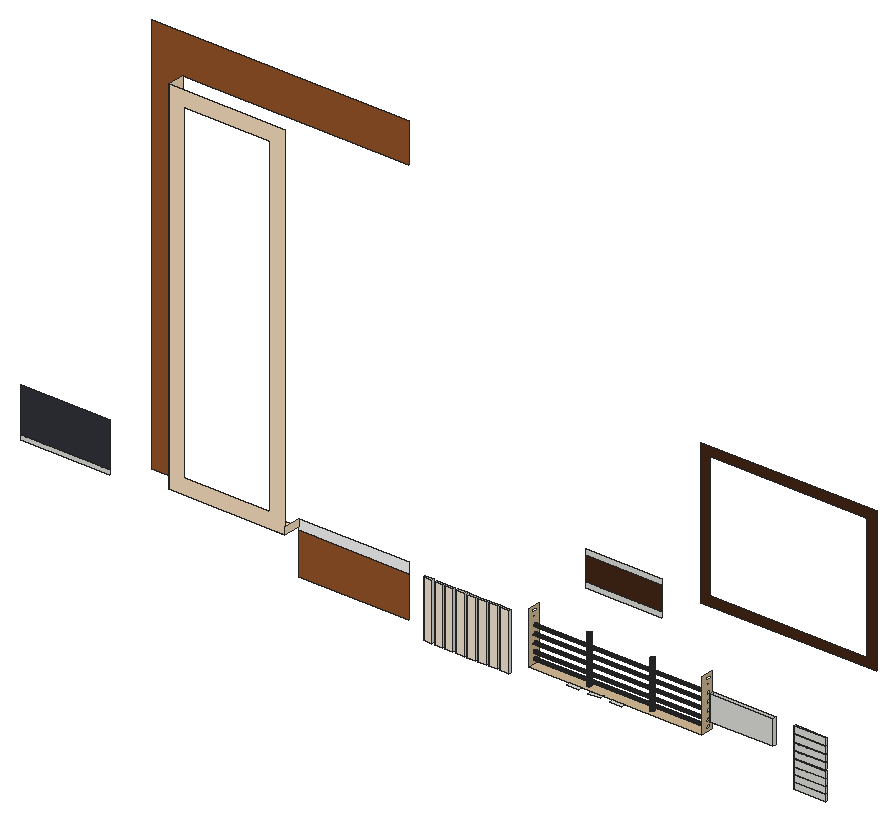
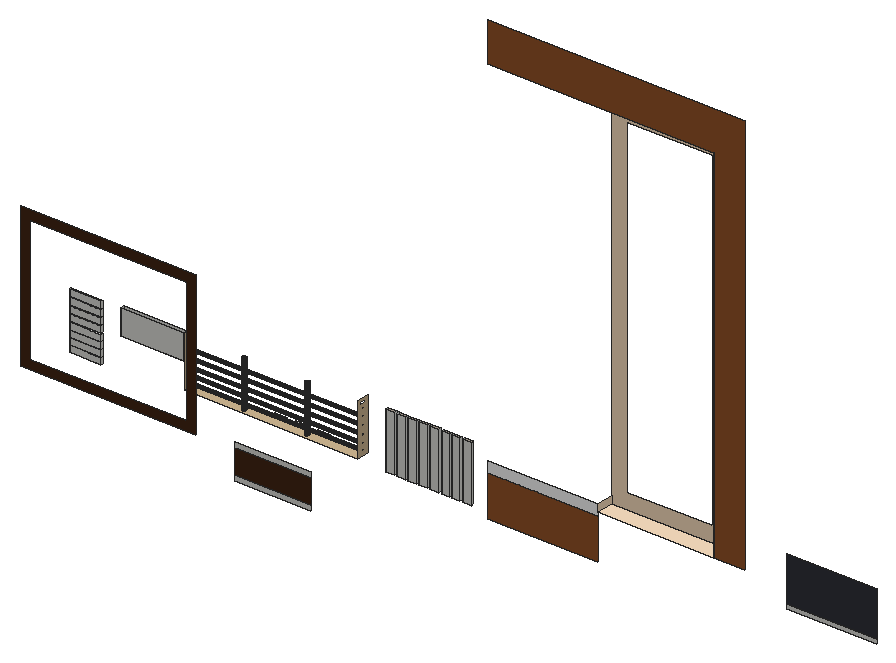
# SketchUp Ruby script. Lengths in inches.
U = 1.inch
M = Sketchup.active_model
def pt(a) = Geom::Point3d.new(a.map { |v| v * U })
def face(e, loops, mat)
  f = e.add_face(loops[0].map { |a| pt(a) })
  loops[1..].each { |l| e.add_face(l.map { |a| pt(a) }).erase! }
  f.material = f.back_material = mat if mat
  f
end
# faces: each face lists its corners as indices into pts; further lists are holes
def faces(e, pts, list, mat = nil) = list.each { |f| face(e, (f[0].is_a?(Array) ? f : [f]).map { |l| l.map { |i| pts[i] } }, mat) }
# xy, xz, yz: faces in a plane at the given z, y or x. An outline is a flat list of corners, or four numbers for a rectangle; further outlines are holes
def ring(l) = l.size == 4 ? [[l[0], l[1]], [l[2], l[1]], [l[2], l[3]], [l[0], l[3]]] : l.each_slice(2).to_a
def flat(e, list, mat, &to3) = list.each { |f| face(e, (f[0].is_a?(Array) ? f : [f]).map { |l| ring(l).map { |u, v| to3.(u, v) } }, mat) }
def xy(e, z, list, mat = nil) = flat(e, list, mat) { |x, y| [x, y, z] }
def xz(e, y, list, mat = nil) = flat(e, list, mat) { |x, z| [x, y, z] }
def yz(e, x, list, mat = nil) = flat(e, list, mat) { |y, z| [x, y, z] }
def lines(e, pts, list) = list.each { |a, b| e.add_line(pt(pts[a]), pt(pts[b])) }
# prism: a flat outline (further loops are holes) pulled along v
def prism(e, loops, v, mat = nil)
  f = face(e, loops, mat); d = Geom::Vector3d.new(v.map { |x| x * U })
  f.pushpull(f.normal.samedirection?(d) ? d.length : -d.length)
end
def box(e, o, s, mat = nil) = prism(e, [[o, [o[0] + s[0], o[1], o[2]], [o[0] + s[0], o[1] + s[1], o[2]], [o[0], o[1] + s[1], o[2]]]], [0, 0, s[2]], mat)
def at(x, y, z, deg = 0) = Geom::Transformation.translation(pt([x, y, z])) * Geom::Transformation.rotation(ORIGIN, Z_AXIS, deg.degrees)
def axes(o, x, y, z) = Geom::Transformation.new([*x, 0, *y, 0, *z, 0, *pt(o).to_a, 1])
def part(name) = M.definitions.add(name)
# library, detail: a bought-in or finely detailed component or shape, given as its bounding box
def library(name, o, s) = part(name).tap { |d| box(d.entities, o, s) }
def detail(e, o, s) = box(e.add_group.entities, o, s)
def put(e, d, t, mat = nil) = e.add_instance(d, t).tap { |i| i.material = mat if mat }
def group(e, t, mat = nil) = e.add_group.tap { |g| g.transformation = t; g.material = mat if mat }.entities
root = M.entities
M.materials.add("[0012_Bisque]").color = [255, 228, 196]
M.materials.add("[0028_AntiqueWhite]").color = [250, 235, 215]
M.materials.add("[Color M00]").color = [255, 255, 255]
M.materials.add("[Color M08]").color = [30, 30, 30]
M.materials.add("[Formica Beige]").color = [211, 187, 149]
M.materials.add("[Formica Laminate Dark]").color = [50, 53, 60]
M.materials.add("[Wood Cherry Original]").color = [152, 86, 42]
M.materials.add("[Wood Veneer 01]").color = [68, 40, 21]
box(root,[409.2,39.8,138.47],[15.5,0.87,3.18])
box(root,[409.2,39.8,141.72],[15.5,0.87,3.18])
box(root,[409.2,39.8,145.15],[15.5,0.87,3.19])
box(root,[409.2,39.8,148.53],[15.5,0.87,3.19])
box(root,[409.2,39.8,152.34],[15.5,0.87,3.19])
box(root,[409.2,39.8,155.84],[15.5,0.87,3.19])
box(root,[409.2,39.8,159.47],[15.5,0.87,3.18])
xy(root,140.39,[[227.93,39.48,232.05,40.67],[233.37,39.48,237.49,40.67],[238.43,39.48,242.55,40.67],[244.05,39.48,248.18,40.67],[249.43,39.48,253.55,40.67],
  [254.74,39.48,258.87,40.67],[260.12,39.48,264.24,40.67],[265.49,39.48,269.62,40.67]])
xy(root,145.875,[[298.64,38.8,304.69,40.67],[309.14,38.8,315.19,40.67],[319.64,38.8,325.69,40.67],[336.54,43.14,336.28,43.17,336.04,43.27,335.83,43.43,335.67,43.64,335.57,43.88,335.54,44.14,335.57,44.4,335.67,44.64,335.83,44.85,336.04,45.01,336.28,45.11,336.54,45.14,336.79,45.11,337.04,45.01,337.24,44.85,337.4,44.64,337.5,44.4,337.54,44.14,337.5,43.88,337.4,43.64,337.24,43.43,337.04,43.27,336.79,43.17]])
xy(root,145.875,[[[278.51,40.67,363.63,46.73],[305.54,43.14,305.28,43.17,305.04,43.27,304.83,43.43,304.67,43.64,304.57,43.88,304.54,44.14,304.57,44.4,304.67,44.64,304.83,44.85,305.04,45.01,305.28,45.11,305.54,45.14,305.79,45.11,306.04,45.01,306.24,44.85,306.4,44.64,306.5,44.4,306.54,44.14,306.5,43.88,306.4,43.64,306.24,43.43,306.04,43.27,305.79,43.17],[336.54,43.14,336.28,43.17,336.04,43.27,335.83,43.43,335.67,43.64,335.57,43.88,335.54,44.14,335.57,44.4,335.67,44.64,335.83,44.85,336.04,45.01,336.28,45.11,336.54,45.14,336.79,45.11,337.04,45.01,337.24,44.85,337.4,44.64,337.5,44.4,337.54,44.14,337.5,43.88,337.4,43.64,337.24,43.43,337.04,43.27,336.79,43.17]]],"[Formica Beige]")
xy(root,154.46,[[368.61,38.8,399.74,40.67]])
xy(root,163.09,[[409.2,39.8,424.7,40.67]])
xy(root,163.67,[[104.08,38.36,161.14,46.73]],"[0012_Bisque]")
xz(root,38.36,[[[104.08,163.67,161.14,341.36],[111.55,171.14,153.67,333.89]]],"[0012_Bisque]")
xz(root,38.8,[[368.61,154.46,399.74,166.58]])
xz(root,39.48,[[227.93,140.39,232.05,168.02],[233.37,140.39,237.49,168.02],[238.43,140.39,242.55,168.02],[244.05,140.39,248.18,168.02],[249.43,140.39,253.55,168.02],
  [254.74,140.39,258.87,168.02],[260.12,140.39,264.24,168.02],[265.49,140.39,269.62,168.02]],"[0028_AntiqueWhite]")
xz(root,39.8,[[409.2,163.09,424.7,166.28]])
xz(root,40.67,[[227.93,140.39,232.05,168.02],[233.37,140.39,237.49,168.02],[238.43,140.39,242.55,168.02],[244.05,140.39,248.18,168.02],[249.43,140.39,253.55,168.02],
  [254.74,140.39,258.87,168.02],[260.12,140.39,264.24,168.02],[265.49,140.39,269.62,168.02],[368.61,154.46,399.74,166.58],[409.2,163.09,424.7,166.28]])
xz(root,46.73,[[24.6875,153.73,68.38,156.02]])
xz(root,46.73,[[161.14,161.98,215,167.14]],"[Color M00]")
xz(root,46.73,[[24.6875,156.02,68.38,177.73]],"[Formica Laminate Dark]")
xz(root,46.73,[[161.14,141.51,215,161.98],[89.06,163.67,104.08,163.67,104.08,341.36,215,341.36,215,360.6,89.06,360.6]],"[Wood Cherry Original]")
xz(root,96.17,[[262.03,150.42,299.47,153.01],[262.03,164.92,299.47,167.51]])
xz(root,96.17,[[262.03,153.01,299.47,164.92],[[318.53,163.84,404.47,234.09],[323.03,168.34,399.97,229.59]]],"[Wood Veneer 01]")
yz(root,104.08,[[38.36,163.67,46.73,341.36]],"[0012_Bisque]")
yz(root,161.14,[[38.36,163.67,46.73,167.14]],"[0012_Bisque]")
yz(root,227.93,[[39.48,140.39,40.67,168.02]])
yz(root,232.05,[[39.48,140.39,40.67,168.02]])
yz(root,233.37,[[39.48,140.39,40.67,168.02]])
yz(root,237.49,[[39.48,140.39,40.67,168.02]])
yz(root,238.43,[[39.48,140.39,40.67,168.02]])
yz(root,242.55,[[39.48,140.39,40.67,168.02]])
yz(root,244.05,[[39.48,140.39,40.67,168.02]])
yz(root,248.18,[[39.48,140.39,40.67,168.02]])
yz(root,249.43,[[39.48,140.39,40.67,168.02]])
yz(root,253.55,[[39.48,140.39,40.67,168.02]])
yz(root,254.74,[[39.48,140.39,40.67,168.02]])
yz(root,258.87,[[39.48,140.39,40.67,168.02]])
yz(root,260.12,[[39.48,140.39,40.67,168.02]])
yz(root,264.24,[[39.48,140.39,40.67,168.02]])
yz(root,265.49,[[39.48,140.39,40.67,168.02]])
yz(root,269.62,[[39.48,140.39,40.67,168.02]])
yz(root,278.51,[[[40.67,145.875,46.73,171.25],[42.95,168.7,45.58,170.07],[43.9,166.34,43.74,166.37,43.59,166.4375,43.47,166.54,43.37,166.68,43.3125,166.83,43.3,166.99,43.33,167.15,43.39,167.3,43.5,167.43,43.63,167.52,43.78,167.58,43.94,167.59,44.11,167.57,44.25,167.5,44.38,167.4,44.47,167.26,44.53,167.11,44.55,166.95,44.52,166.79,44.45,166.64,44.35,166.51,44.22,166.42,44.06,166.36],[43.9,162.53,43.74,162.56,43.59,162.625,43.47,162.73,43.37,162.86,43.3125,163.02,43.3,163.18,43.33,163.34,43.39,163.49,43.5,163.61,43.63,163.71,43.78,163.77,43.94,163.78,44.11,163.76,44.25,163.6875,44.38,163.58,44.47,163.45,44.53,163.3,44.55,163.14,44.52,162.97,44.45,162.83,44.35,162.7,44.22,162.61,44.06,162.55],[43.9,158.53,43.74,158.56,43.59,158.625,43.47,158.73,43.37,158.86,43.3125,159.02,43.3,159.18,43.33,159.34,43.39,159.49,43.5,159.61,43.63,159.71,43.78,159.77,43.94,159.78,44.11,159.76,44.25,159.6875,44.38,159.58,44.47,159.45,44.53,159.3,44.55,159.14,44.52,158.97,44.45,158.83,44.35,158.7,44.22,158.61,44.06,158.55],[43.9,154.53,43.74,154.56,43.59,154.625,43.47,154.73,43.37,154.86,43.3125,155.02,43.3,155.18,43.33,155.34,43.39,155.49,43.5,155.61,43.63,155.71,43.78,155.77,43.94,155.78,44.11,155.76,44.25,155.6875,44.38,155.58,44.47,155.45,44.53,155.3,44.55,155.14,44.52,154.97,44.45,154.83,44.35,154.7,44.22,154.61,44.06,154.55],[43.9,147.66,43.74,147.68,43.59,147.75,43.47,147.86,43.37,147.99,43.3125,148.14,43.3,148.3,43.33,148.46,43.39,148.61,43.5,148.74,43.63,148.83,43.78,148.89,43.94,148.91,44.11,148.88,44.25,148.8125,44.38,148.71,44.47,148.58,44.53,148.42,44.55,148.26,44.52,148.1,44.45,147.95,44.35,147.83,44.22,147.73,44.06,147.67],[43.9,150.84,43.74,150.87,43.59,150.9375,43.47,151.04,43.37,151.18,43.3125,151.33,43.3,151.49,43.33,151.65,43.39,151.8,43.5,151.93,43.63,152.02,43.78,152.08,43.94,152.09,44.11,152.07,44.25,152,44.38,151.9,44.47,151.76,44.53,151.61,44.55,151.45,44.52,151.29,44.45,151.14,44.35,151.01,44.22,150.92,44.06,150.86]]],"[Formica Beige]")
yz(root,363.63,[[43.9,147.66,44.06,147.67,44.22,147.73,44.35,147.83,44.45,147.95,44.52,148.1,44.55,148.26,44.53,148.42,44.47,148.58,44.38,148.71,44.25,148.8125,44.11,148.88,43.94,148.91,43.78,148.89,43.63,148.83,43.5,148.74,43.39,148.61,43.33,148.46,43.3,148.3,43.3125,148.14,43.37,147.99,43.47,147.86,43.59,147.75,43.74,147.68],[43.9,150.84,44.06,150.86,44.22,150.92,44.35,151.01,44.45,151.14,44.52,151.29,44.55,151.45,44.53,151.61,44.47,151.76,44.38,151.9,44.25,152,44.11,152.07,43.94,152.09,43.78,152.08,43.63,152.02,43.5,151.93,43.39,151.8,43.33,151.65,43.3,151.49,43.3125,151.33,43.37,151.18,43.47,151.04,43.59,150.9375,43.74,150.87],[43.9,154.53,44.06,154.55,44.22,154.61,44.35,154.7,44.45,154.83,44.52,154.97,44.55,155.14,44.53,155.3,44.47,155.45,44.38,155.58,44.25,155.6875,44.11,155.76,43.94,155.78,43.78,155.77,43.63,155.71,43.5,155.61,43.39,155.49,43.33,155.34,43.3,155.18,43.3125,155.02,43.37,154.86,43.47,154.73,43.59,154.625,43.74,154.56],[43.9,158.53,44.06,158.55,44.22,158.61,44.35,158.7,44.45,158.83,44.52,158.97,44.55,159.14,44.53,159.3,44.47,159.45,44.38,159.58,44.25,159.6875,44.11,159.76,43.94,159.78,43.78,159.77,43.63,159.71,43.5,159.61,43.39,159.49,43.33,159.34,43.3,159.18,43.3125,159.02,43.37,158.86,43.47,158.73,43.59,158.625,43.74,158.56],[43.9,162.53,44.06,162.55,44.22,162.61,44.35,162.7,44.45,162.83,44.52,162.97,44.55,163.14,44.53,163.3,44.47,163.45,44.38,163.58,44.25,163.6875,44.11,163.76,43.94,163.78,43.78,163.77,43.63,163.71,43.5,163.61,43.39,163.49,43.33,163.34,43.3,163.18,43.3125,163.02,43.37,162.86,43.47,162.73,43.59,162.625,43.74,162.56]])
yz(root,363.63,[[[40.67,145.875,46.73,171.25],[42.95,168.7,45.58,170.07],[43.9,166.34,44.06,166.36,44.22,166.42,44.35,166.51,44.45,166.64,44.52,166.79,44.55,166.95,44.53,167.11,44.47,167.26,44.38,167.4,44.25,167.5,44.11,167.57,43.94,167.59,43.78,167.58,43.63,167.52,43.5,167.43,43.39,167.3,43.33,167.15,43.3,166.99,43.3125,166.83,43.37,166.68,43.47,166.54,43.59,166.4375,43.74,166.37],[43.9,147.66,44.06,147.67,44.22,147.73,44.35,147.83,44.45,147.95,44.52,148.1,44.55,148.26,44.53,148.42,44.47,148.58,44.38,148.71,44.25,148.8125,44.11,148.88,43.94,148.91,43.78,148.89,43.63,148.83,43.5,148.74,43.39,148.61,43.33,148.46,43.3,148.3,43.3125,148.14,43.37,147.99,43.47,147.86,43.59,147.75,43.74,147.68],[43.9,162.53,44.06,162.55,44.22,162.61,44.35,162.7,44.45,162.83,44.52,162.97,44.55,163.14,44.53,163.3,44.47,163.45,44.38,163.58,44.25,163.6875,44.11,163.76,43.94,163.78,43.78,163.77,43.63,163.71,43.5,163.61,43.39,163.49,43.33,163.34,43.3,163.18,43.3125,163.02,43.37,162.86,43.47,162.73,43.59,162.625,43.74,162.56],[43.9,150.84,44.06,150.86,44.22,150.92,44.35,151.01,44.45,151.14,44.52,151.29,44.55,151.45,44.53,151.61,44.47,151.76,44.38,151.9,44.25,152,44.11,152.07,43.94,152.09,43.78,152.08,43.63,152.02,43.5,151.93,43.39,151.8,43.33,151.65,43.3,151.49,43.3125,151.33,43.37,151.18,43.47,151.04,43.59,150.9375,43.74,150.87],[43.9,158.53,44.06,158.55,44.22,158.61,44.35,158.7,44.45,158.83,44.52,158.97,44.55,159.14,44.53,159.3,44.47,159.45,44.38,159.58,44.25,159.6875,44.11,159.76,43.94,159.78,43.78,159.77,43.63,159.71,43.5,159.61,43.39,159.49,43.33,159.34,43.3,159.18,43.3125,159.02,43.37,158.86,43.47,158.73,43.59,158.625,43.74,158.56],[43.9,154.53,44.06,154.55,44.22,154.61,44.35,154.7,44.45,154.83,44.52,154.97,44.55,155.14,44.53,155.3,44.47,155.45,44.38,155.58,44.25,155.6875,44.11,155.76,43.94,155.78,43.78,155.77,43.63,155.71,43.5,155.61,43.39,155.49,43.33,155.34,43.3,155.18,43.3125,155.02,43.37,154.86,43.47,154.73,43.59,154.625,43.74,154.56]]],"[Formica Beige]")
yz(root,368.61,[[38.8,154.46,40.67,166.58]])
yz(root,399.74,[[38.8,154.46,40.67,166.58]])
yz(root,409.2,[[39.8,163.09,40.67,166.28]])
yz(root,424.7,[[39.8,163.09,40.67,166.28]])
p = [[305.28,43.17,145.875],[305.54,43.14,145.875],[305.54,43.14,168.8125],[305.28,43.17,168.8125],[305.79,43.17,145.875],[305.79,43.17,168.8125],
  [336.28,43.17,145.875],[336.54,43.14,145.875],[336.54,43.14,168.7],[336.28,43.17,168.7],[336.79,43.17,145.875],[336.79,43.17,168.7],
  [305.04,43.27,145.875],[305.04,43.27,168.8125],[306.04,43.27,145.875],[306.04,43.27,168.8125],[336.04,43.27,145.875],[336.04,43.27,168.7],
  [337.04,43.27,145.875],[337.04,43.27,168.7],[304.83,43.43,145.875],[304.83,43.43,168.8125],[306.24,43.43,145.875],[306.24,43.43,168.8125],
  [335.83,43.43,145.875],[335.83,43.43,168.7],[337.24,43.43,145.875],[337.24,43.43,168.7],[304.67,43.64,145.875],[304.67,43.64,168.8125],
  [306.4,43.64,145.875],[306.4,43.64,168.8125],[335.67,43.64,145.875],[335.67,43.64,168.7],[337.4,43.64,145.875],[337.4,43.64,168.7],
  [304.57,43.88,145.875],[304.57,43.88,168.8125],[306.5,43.88,145.875],[306.5,43.88,168.8125],[335.57,43.88,145.875],[335.57,43.88,168.7],
  [337.5,43.88,145.875],[337.5,43.88,168.7],[304.54,44.14,145.875],[304.54,44.14,168.8125],[306.54,44.14,145.875],[306.54,44.14,168.8125],
  [335.54,44.14,145.875],[335.54,44.14,168.7],[337.54,44.14,145.875],[337.54,44.14,168.7],[304.57,44.4,145.875],[304.57,44.4,168.8125],
  [306.5,44.4,145.875],[306.5,44.4,168.8125],[335.57,44.4,145.875],[335.57,44.4,168.7],[337.5,44.4,145.875],[337.5,44.4,168.7],
  [304.67,44.64,145.875],[304.67,44.64,168.8125],[306.4,44.64,145.875],[306.4,44.64,168.8125],[335.67,44.64,145.875],[335.67,44.64,168.7],
  [337.4,44.64,145.875],[337.4,44.64,168.7],[304.83,44.85,145.875],[304.83,44.85,168.8125],[306.24,44.85,145.875],[306.24,44.85,168.8125],
  [335.83,44.85,145.875],[335.83,44.85,168.7],[337.24,44.85,145.875],[337.24,44.85,168.7],[305.04,45.01,145.875],[305.04,45.01,168.8125],
  [306.04,45.01,145.875],[306.04,45.01,168.8125],[336.04,45.01,145.875],[336.04,45.01,168.7],[337.04,45.01,145.875],[337.04,45.01,168.7],
  [305.28,45.11,145.875],[305.28,45.11,168.8125],[305.79,45.11,145.875],[305.79,45.11,168.8125],[336.28,45.11,145.875],[336.28,45.11,168.7],
  [336.79,45.11,145.875],[336.79,45.11,168.7],[305.54,45.14,145.875],[305.54,45.14,168.8125],[336.54,45.14,145.875],[336.54,45.14,168.7],
  [363.63,43.74,147.68],[363.63,43.59,147.75],[278.51,43.59,147.75],[278.51,43.74,147.68],[363.63,43.9,147.66],[278.51,43.9,147.66],
  [363.63,44.06,147.67],[278.51,44.06,147.67],[363.63,44.22,147.73],[278.51,44.22,147.73],[363.63,44.35,147.83],[278.51,44.35,147.83],
  [363.63,43.47,147.86],[278.51,43.47,147.86],[363.63,44.45,147.95],[278.51,44.45,147.95],[363.63,43.37,147.99],[278.51,43.37,147.99],
  [363.63,43.3125,148.14],[278.51,43.3125,148.14],[363.63,44.52,148.1],[278.51,44.52,148.1],[363.63,43.3,148.3],[278.51,43.3,148.3],
  [363.63,44.55,148.26],[278.51,44.55,148.26],[363.63,43.33,148.46],[278.51,43.33,148.46],[363.63,44.53,148.42],[278.51,44.53,148.42],
  [363.63,44.47,148.58],[278.51,44.47,148.58],[363.63,43.39,148.61],[278.51,43.39,148.61],[363.63,43.5,148.74],[278.51,43.5,148.74],
  [363.63,44.38,148.71],[278.51,44.38,148.71],[363.63,43.63,148.83],[278.51,43.63,148.83],[363.63,44.25,148.8125],[278.51,44.25,148.8125],
  [363.63,43.78,148.89],[278.51,43.78,148.89],[363.63,44.11,148.88],[278.51,44.11,148.88],[363.63,43.94,148.91],[278.51,43.94,148.91],
  [363.63,43.9,150.84],[363.63,43.74,150.87],[278.51,43.74,150.87],[278.51,43.9,150.84],[363.63,44.06,150.86],[278.51,44.06,150.86],
  [363.63,43.59,150.9375],[363.63,43.47,151.04],[278.51,43.47,151.04],[278.51,43.59,150.9375],[363.63,44.22,150.92],[278.51,44.22,150.92],
  [363.63,44.35,151.01],[278.51,44.35,151.01],[363.63,43.37,151.18],[278.51,43.37,151.18],[363.63,44.45,151.14],[278.51,44.45,151.14],
  [363.63,44.52,151.29],[278.51,44.52,151.29],[363.63,43.3125,151.33],[278.51,43.3125,151.33],[363.63,43.3,151.49],[278.51,43.3,151.49],
  [363.63,44.55,151.45],[278.51,44.55,151.45],[363.63,44.53,151.61],[278.51,44.53,151.61],[363.63,43.33,151.65],[278.51,43.33,151.65],
  [363.63,44.47,151.76],[278.51,44.47,151.76],[363.63,43.39,151.8],[278.51,43.39,151.8],[363.63,43.5,151.93],[278.51,43.5,151.93],
  [363.63,44.38,151.9],[278.51,44.38,151.9],[363.63,43.63,152.02],[278.51,43.63,152.02],[363.63,44.25,152],[278.51,44.25,152],
  [363.63,43.78,152.08],[278.51,43.78,152.08],[363.63,44.11,152.07],[278.51,44.11,152.07],[363.63,43.94,152.09],[278.51,43.94,152.09],
  [363.63,43.9,154.53],[363.63,43.74,154.56],[278.51,43.74,154.56],[278.51,43.9,154.53],[363.63,44.06,154.55],[278.51,44.06,154.55],
  [363.63,44.22,154.61],[278.51,44.22,154.61],[363.63,43.59,154.625],[363.63,43.47,154.73],[278.51,43.47,154.73],[278.51,43.59,154.625],
  [363.63,44.35,154.7],[278.51,44.35,154.7],[363.63,43.37,154.86],[278.51,43.37,154.86],[363.63,44.45,154.83],[278.51,44.45,154.83],
  [363.63,44.52,154.97],[278.51,44.52,154.97],[363.63,43.3125,155.02],[278.51,43.3125,155.02],[363.63,43.3,155.18],[278.51,43.3,155.18],
  [363.63,44.55,155.14],[278.51,44.55,155.14],[363.63,44.53,155.3],[278.51,44.53,155.3],[363.63,43.33,155.34],[278.51,43.33,155.34],
  [363.63,43.39,155.49],[278.51,43.39,155.49],[363.63,44.47,155.45],[278.51,44.47,155.45],[363.63,43.5,155.61],[278.51,43.5,155.61],
  [363.63,44.38,155.58],[278.51,44.38,155.58],[363.63,43.63,155.71],[278.51,43.63,155.71],[363.63,44.25,155.6875],[278.51,44.25,155.6875],
  [363.63,43.78,155.77],[278.51,43.78,155.77],[363.63,44.11,155.76],[278.51,44.11,155.76],[363.63,43.94,155.78],[278.51,43.94,155.78],
  [363.63,43.9,158.53],[363.63,43.74,158.56],[278.51,43.74,158.56],[278.51,43.9,158.53],[363.63,44.06,158.55],[278.51,44.06,158.55],
  [363.63,44.22,158.61],[278.51,44.22,158.61],[363.63,43.59,158.625],[363.63,43.47,158.73],[278.51,43.47,158.73],[278.51,43.59,158.625],
  [363.63,44.35,158.7],[278.51,44.35,158.7],[363.63,43.37,158.86],[278.51,43.37,158.86],[363.63,44.45,158.83],[278.51,44.45,158.83],
  [363.63,44.52,158.97],[278.51,44.52,158.97],[363.63,43.3125,159.02],[278.51,43.3125,159.02],[363.63,43.3,159.18],[278.51,43.3,159.18],
  [363.63,44.55,159.14],[278.51,44.55,159.14],[363.63,44.53,159.3],[278.51,44.53,159.3],[363.63,43.33,159.34],[278.51,43.33,159.34],
  [363.63,43.39,159.49],[278.51,43.39,159.49],[363.63,44.47,159.45],[278.51,44.47,159.45],[363.63,43.5,159.61],[278.51,43.5,159.61],
  [363.63,44.38,159.58],[278.51,44.38,159.58],[363.63,43.63,159.71],[278.51,43.63,159.71],[363.63,44.25,159.6875],[278.51,44.25,159.6875],
  [363.63,43.78,159.77],[278.51,43.78,159.77],[363.63,44.11,159.76],[278.51,44.11,159.76],[363.63,43.94,159.78],[278.51,43.94,159.78],
  [363.63,43.9,162.53],[363.63,43.74,162.56],[278.51,43.74,162.56],[278.51,43.9,162.53],[363.63,44.06,162.55],[278.51,44.06,162.55],
  [363.63,44.22,162.61],[278.51,44.22,162.61],[363.63,43.59,162.625],[363.63,43.47,162.73],[278.51,43.47,162.73],[278.51,43.59,162.625],
  [363.63,44.35,162.7],[278.51,44.35,162.7],[363.63,43.37,162.86],[278.51,43.37,162.86],[363.63,44.45,162.83],[278.51,44.45,162.83],
  [363.63,44.52,162.97],[278.51,44.52,162.97],[363.63,43.3125,163.02],[278.51,43.3125,163.02],[363.63,43.3,163.18],[278.51,43.3,163.18],
  [363.63,44.55,163.14],[278.51,44.55,163.14],[363.63,44.53,163.3],[278.51,44.53,163.3],[363.63,43.33,163.34],[278.51,43.33,163.34],
  [363.63,43.39,163.49],[278.51,43.39,163.49],[363.63,44.47,163.45],[278.51,44.47,163.45],[363.63,43.5,163.61],[278.51,43.5,163.61],
  [363.63,44.38,163.58],[278.51,44.38,163.58],[363.63,43.63,163.71],[278.51,43.63,163.71],[363.63,44.25,163.6875],[278.51,44.25,163.6875],
  [363.63,43.78,163.77],[278.51,43.78,163.77],[363.63,44.11,163.76],[278.51,44.11,163.76],[363.63,43.94,163.78],[278.51,43.94,163.78]]
faces(root,p,[[0,1,2,3],[1,4,5,2],[6,7,8,9],[7,10,11,8],[12,0,3,13],[4,14,15,5],[16,6,9,17],[10,18,19,11],
  [20,12,13,21],[14,22,23,15],[24,16,17,25],[18,26,27,19],[28,20,21,29],[22,30,31,23],[32,24,25,33],[26,34,35,27],
  [36,28,29,37],[30,38,39,31],[40,32,33,41],[34,42,43,35],[44,36,37,45],[38,46,47,39],[48,40,41,49],[42,50,51,43],
  [52,44,45,53],[46,54,55,47],[56,48,49,57],[50,58,59,51],[60,52,53,61],[54,62,63,55],[64,56,57,65],[58,66,67,59],
  [68,60,61,69],[62,70,71,63],[72,64,65,73],[66,74,75,67],[76,68,69,77],[70,78,79,71],[80,72,73,81],[74,82,83,75],
  [84,76,77,85],[78,86,87,79],[88,80,81,89],[82,90,91,83],[92,84,85,93],[86,92,93,87],[94,88,89,95],[90,94,95,91],
  [96,97,98,99],[100,96,99,101],[102,100,101,103],[104,102,103,105],[106,104,105,107],[97,108,109,98],[110,106,107,111],[108,112,113,109],
  [112,114,115,113],[116,110,111,117],[114,118,119,115],[120,116,117,121],[118,122,123,119],[124,120,121,125],[126,124,125,127],[122,128,129,123],
  [128,130,131,129],[132,126,127,133],[130,134,135,131],[136,132,133,137],[134,138,139,135],[140,136,137,141],[138,142,143,139],[142,140,141,143],
  [144,145,146,147],[148,144,147,149],[150,151,152,153],[145,150,153,146],[154,148,149,155],[156,154,155,157],[151,158,159,152],[160,156,157,161],
  [162,160,161,163],[158,164,165,159],[164,166,167,165],[168,162,163,169],[170,168,169,171],[166,172,173,167],[174,170,171,175],[172,176,177,173],
  [176,178,179,177],[180,174,175,181],[178,182,183,179],[184,180,181,185],[182,186,187,183],[188,184,185,189],[186,190,191,187],[190,188,189,191],
  [192,193,194,195],[196,192,195,197],[198,196,197,199],[200,201,202,203],[193,200,203,194],[204,198,199,205],[201,206,207,202],[208,204,205,209],
  [210,208,209,211],[206,212,213,207],[212,214,215,213],[216,210,211,217],[218,216,217,219],[214,220,221,215],[220,222,223,221],[224,218,219,225],
  [222,226,227,223],[228,224,225,229],[226,230,231,227],[232,228,229,233],[230,234,235,231],[236,232,233,237],[234,238,239,235],[238,236,237,239],
  [240,241,242,243],[244,240,243,245],[246,244,245,247],[248,249,250,251],[241,248,251,242],[252,246,247,253],[249,254,255,250],[256,252,253,257],
  [258,256,257,259],[254,260,261,255],[260,262,263,261],[264,258,259,265],[266,264,265,267],[262,268,269,263],[268,270,271,269],[272,266,267,273],
  [270,274,275,271],[276,272,273,277],[274,278,279,275],[280,276,277,281],[278,282,283,279],[284,280,281,285],[282,286,287,283],[286,284,285,287],
  [288,289,290,291],[292,288,291,293],[294,292,293,295],[296,297,298,299],[289,296,299,290],[300,294,295,301],[297,302,303,298],[304,300,301,305],
  [306,304,305,307],[302,308,309,303],[308,310,311,309],[312,306,307,313],[314,312,313,315],[310,316,317,311],[316,318,319,317],[320,314,315,321],
  [318,322,323,319],[324,320,321,325],[322,326,327,323],[328,324,325,329],[326,330,331,327],[332,328,329,333],[330,334,335,331],[334,332,333,335]],"[Color M08]")
